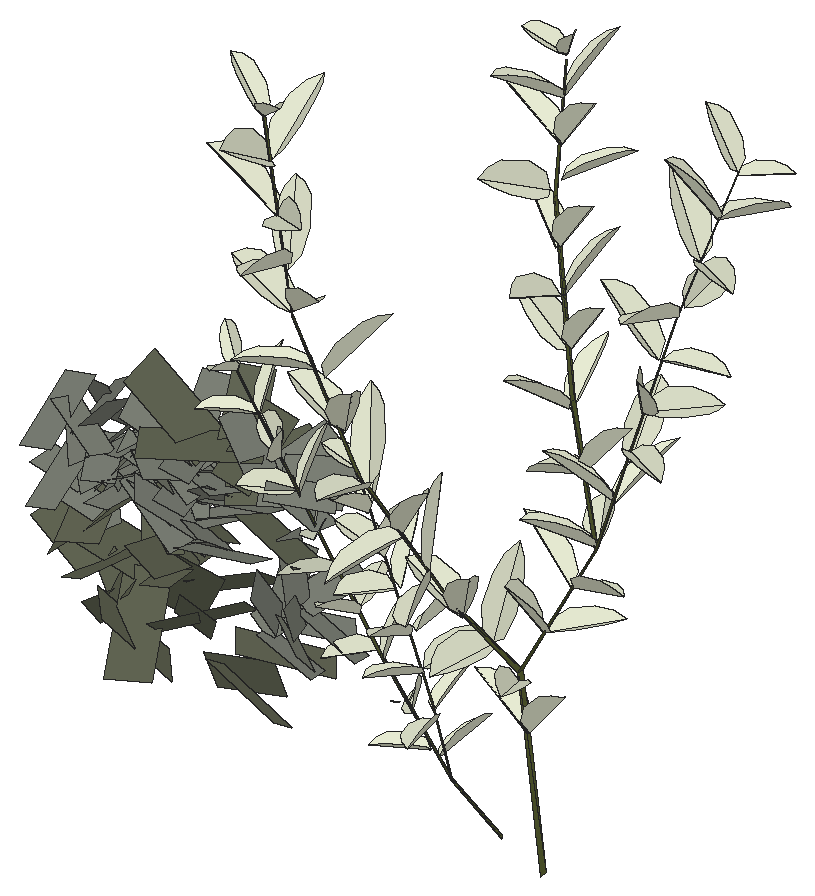
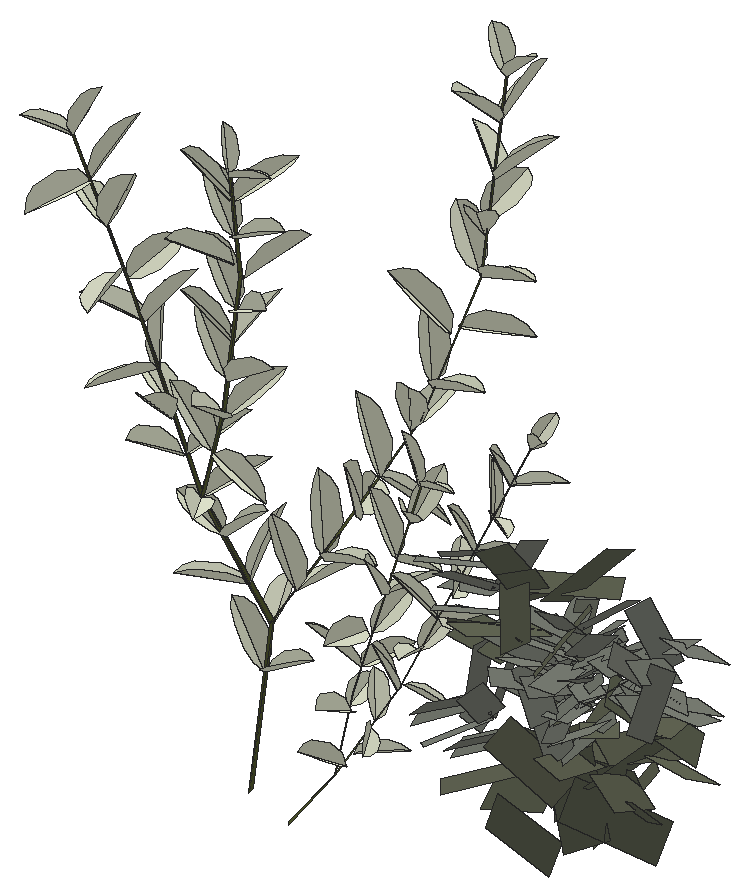
# SketchUp Ruby script. Lengths in inches.
U = 1.inch
M = Sketchup.active_model
def pt(a) = Geom::Point3d.new(a.map { |v| v * U })
def face(e, loops, mat)
  f = e.add_face(loops[0].map { |a| pt(a) })
  loops[1..].each { |l| e.add_face(l.map { |a| pt(a) }).erase! }
  f.material = f.back_material = mat if mat
  f
end
# faces: each face lists its corners as indices into pts; further lists are holes
def faces(e, pts, list, mat = nil) = list.each { |f| face(e, (f[0].is_a?(Array) ? f : [f]).map { |l| l.map { |i| pts[i] } }, mat) }
# xy, xz, yz: faces in a plane at the given z, y or x. An outline is a flat list of corners, or four numbers for a rectangle; further outlines are holes
def ring(l) = l.size == 4 ? [[l[0], l[1]], [l[2], l[1]], [l[2], l[3]], [l[0], l[3]]] : l.each_slice(2).to_a
def flat(e, list, mat, &to3) = list.each { |f| face(e, (f[0].is_a?(Array) ? f : [f]).map { |l| ring(l).map { |u, v| to3.(u, v) } }, mat) }
def xy(e, z, list, mat = nil) = flat(e, list, mat) { |x, y| [x, y, z] }
def xz(e, y, list, mat = nil) = flat(e, list, mat) { |x, z| [x, y, z] }
def yz(e, x, list, mat = nil) = flat(e, list, mat) { |y, z| [x, y, z] }
def lines(e, pts, list) = list.each { |a, b| e.add_line(pt(pts[a]), pt(pts[b])) }
# prism: a flat outline (further loops are holes) pulled along v
def prism(e, loops, v, mat = nil)
  f = face(e, loops, mat); d = Geom::Vector3d.new(v.map { |x| x * U })
  f.pushpull(f.normal.samedirection?(d) ? d.length : -d.length)
end
def box(e, o, s, mat = nil) = prism(e, [[o, [o[0] + s[0], o[1], o[2]], [o[0] + s[0], o[1] + s[1], o[2]], [o[0], o[1] + s[1], o[2]]]], [0, 0, s[2]], mat)
def at(x, y, z, deg = 0) = Geom::Transformation.translation(pt([x, y, z])) * Geom::Transformation.rotation(ORIGIN, Z_AXIS, deg.degrees)
def axes(o, x, y, z) = Geom::Transformation.new([*x, 0, *y, 0, *z, 0, *pt(o).to_a, 1])
def part(name) = M.definitions.add(name)
# library, detail: a bought-in or finely detailed component or shape, given as its bounding box
def library(name, o, s) = part(name).tap { |d| box(d.entities, o, s) }
def detail(e, o, s) = box(e.add_group.entities, o, s)
def put(e, d, t, mat = nil) = e.add_instance(d, t).tap { |i| i.material = mat if mat }
def group(e, t, mat = nil) = e.add_group.tap { |g| g.transformation = t; g.material = mat if mat }.entities
root = M.entities
M.materials.add("0ad16as01f6asdLeafVar1sfd015as60f1as6").color = [231, 235, 211]
M.materials.add("asdfasdf0165f6asdLeafVar1sfd015as60f1as6").color = [231, 235, 211]
M.materials.add("dw_stemssadfasdfa0sdf1s01d6w1").color = [90, 97, 50]
M.materials.add("viburnumblaasdfas0df1w06d").color = [98, 102, 84]
M.materials.add("viburnumbladsadfasdfad0w122").color = [125, 129, 119]
c1 = part("Component\#315")
p = [[0.25,0,0],[2.05,0.01,0.35],[1.81,4.2,1.66],[0,4.19,1.3125]]
faces(c1.entities,p,[[0,1,2,3]],"viburnumbladsadfasdfad0w122")
c2 = part("viburnumblad2")
put(c2.entities,c1,axes([-19.23,-4.49,-32.18],[83.35428,0,0],[0,79.38502,0],[0,0,83.35428]))
c3 = part("Component\#314")
p = [[0.14,0,0],[2.58,0.05,0.25],[2.44,5.11,2.64],[0,5.05,2.39]]
faces(c3.entities,p,[[0,1,2,3]],"viburnumblaasdfas0df1w06d")
c4 = part("viburnumblad1\#2")
put(c4.entities,c3,axes([-37.25,6.23,19.31],[75.98784,0,0],[0,65.50676,0],[0,0,75.98784]))
c5 = part("vdw_leaf\#1")
p = [[0,0,0],[-2.77,1.61,2.32],[-4.3125,6.1,4.5],[-3.97,13.49,6.09],[-2.47,18.57,6.3],[-0.2,22.73,5.75],
  [2.54,19.66,6.85],[4.3,15.93,7.09],[5.03,7.6,5.43],[3.32,1.76,2.74]]
faces(c5.entities,p,[[0,1,2,3,4,5],[0,5,6,7,8,9]],"0ad16as01f6asdLeafVar1sfd015as60f1as6")
c6 = part("dw_branch_3\#2")
p = [[-10.06,-1.6,62.9],[-0.2,1.54,-0.01],[-10.43,1.54,62.72],[0.18,-1.6,0.17],[-23.75,-21.66,88.91],[-25.7,-20.3,89.55],
  [13.4,11.62,104.56],[13.33,13.52,104.47],[-49.25,-41.87,130.3125],[-50.33,-40.21,130.71],[-4.97,21.13,143.98],[35.61,27.99,178.64],
  [-5.09,23.64,143.96],[35.32,29.14,178.46],[-67.7,-55.38,181.06],[-68.34,-54.45,181.62],[-22.8125,33.9,200.59],[-22.94,35.79,200.41],
  [56.61,36.78,229.75],[56.29,38.09,229.57],[-70.63,-67.46,248.85],[-70.72,-66.33,249.5],[-25.05,43.32,240.75],[-24.98,44.26,240.57]]
faces(c6.entities,p,[[0,1,2],[0,3,1],[4,2,5],[4,0,2],[6,0,2],[6,2,7],[8,4,5],[8,5,9],
  [10,6,7],[11,6,7],[10,7,12],[11,7,13],[14,8,9],[14,9,15],[16,10,12],[16,12,17],
  [18,11,13],[18,13,19],[20,14,15],[20,15,21],[22,16,17],[22,17,23]],"dw_stemssadfasdfa0sdf1s01d6w1")
c7 = part("dw_branch3\#2")
put(c7.entities,c5,axes([-70.33,-63.58,233.32],[-1.00752,0.412,0.78596],[-0.24851,-1.22189,0.32195],[0.83141,0.09817,1.01433]))
put(c7.entities,c5,axes([-66.93,-54.91,182.82],[-0.84976,-0.98359,0.33619],[0.99572,-0.74889,0.32577],[-0.05223,0.46521,1.22907]))
put(c7.entities,c5,axes([-46.12,-39.49,126.35],[1.23843,0.5364,0.23552],[-0.56438,0.94474,0.81599],[0.15707,-0.83465,1.07498]))
put(c7.entities,c5,axes([13.0625,13.13,104.77],[-1.01271,0.69982,-0.26884],[-0.74268,-0.99813,0.19939],[-0.10222,0.31872,1.21473]))
put(c7.entities,c5,axes([-18.87,30.42,186.42],[0.36309,1.06515,-0.56675],[-1.14134,0.49515,0.19939],[0.39128,0.45593,1.10754]))
put(c7.entities,c5,axes([-3.2,4.15,75.77],[-1.04153,0.55414,0.44243],[-0.23365,-1.01045,0.71554],[0.6695,0.50943,0.93801]))
put(c7.entities,c5,axes([23.2,19.41,136.3],[-0.65687,-1.11295,-0.05714],[1.05857,-0.61429,-0.20411],[0.15163,-0.1536,1.24868]))
put(c7.entities,c5,axes([-25.57,35.48,201.32],[-0.64726,0.62827,0.87973],[-0.71635,-1.0172,0.19939],[0.80962,-0.39773,0.87973]))
put(c7.entities,c5,axes([-36.37,-32.14,110.35],[-0.80747,1.09962,0.12544],[-0.83333,-0.50188,-0.96467],[-0.72833,-0.64487,0.96467]))
put(c7.entities,c5,axes([-9.89,26.72,156.79],[0.45529,1.02969,0.56572],[-1.16919,0.33753,0.32662],[0.11537,-0.64297,1.07744]))
put(c7.entities,c5,axes([-26.57,46.1,241.0625],[0.00015,0.80921,0.22536],[-0.83985,0.00446,-0.01542],[-0.01605,-0.22532,0.80906]))
put(c7.entities,c5,axes([-9.2,-2.58,61.06],[-1.10001,-0.40312,0.39014],[0.40883,-1.1116,0.00411],[0.35732,0.13566,1.14763]))
put(c7.entities,c5,axes([-69.91,-63.11,233.93],[1.36249,-0.1432,0],[0.13201,1.25603,0.5309],[-0.05549,-0.52799,1.26295]))
put(c7.entities,c5,axes([32.2,25.46,166.13],[0.06878,-1.29051,-0.05714],[1.22165,0.07415,-0.20411],[0.2113,-0.04403,1.24868]))
put(c7.entities,c5,axes([-5.68,-0.66,44.43],[-0.48448,-1.12287,0.17078],[0.98138,-0.33653,0.57135],[-0.48308,0.36756,1.04626]))
put(c7.entities,c5,axes([43.45,32.81,198.64],[0.5408,1.19584,0.14106],[-0.94242,0.32409,0.86557],[0.74952,-0.45533,0.98656]))
put(c7.entities,c5,axes([12.52,14.14,104.98],[1.02694,0.54888,0.41092],[-0.53566,1.05407,-0.06927],[-0.38969,-0.12321,1.13846]))
put(c7.entities,c5,axes([44.55,32.375,198.73],[-0.65687,-1.11295,-0.05714],[1.05857,-0.61429,-0.20411],[0.15163,-0.1536,1.24868]))
put(c7.entities,c5,axes([-5.67,21.17,141.44],[-1.10726,0.43603,-0.32953],[-0.49537,-1.03435,0.29588],[-0.17521,0.40597,1.12589]))
put(c7.entities,c5,axes([55.69,37.84,229.48],[0.18984,0.96334,0.18958],[-0.71996,0.0053,0.69399],[0.66755,-0.26823,0.69457]))
put(c7.entities,c5,axes([-21.52,36.85,205.2],[0.72606,-0.98817,0.14519],[0.94364,0.7084,0.10251],[-0.16885,0.05176,1.19664]))
put(c7.entities,c5,axes([-68.51,-56.35,196.07],[1.16319,0.72381,0],[-0.66725,1.0723,0.5309],[0.28049,-0.45075,1.26295]))
put(c7.entities,c6,at(0.01,-0.09,-0.02),"dw_stemssadfasdfa0sdf1s01d6w1")
put(c7.entities,c5,axes([-2.49,5.18,75.91],[0.78614,-0.90346,-0.30078],[0.86953,0.79562,-0.11715],[0.28546,-0.14014,1.16705]))
put(c7.entities,c5,axes([-23.125,-16.22,82.25],[0.32175,1.32576,0.12544],[-1.33153,0.31835,0.05068],[0.01989,-0.13382,1.3633]))
put(c7.entities,c5,axes([-23.75,41.99,230.3],[0.85958,-0.87451,0.14519],[0.66531,0.75721,0.62192],[-0.54076,-0.36226,1.01955]))
put(c7.entities,c5,axes([27.07,22.48,149.34],[0.92952,-0.64745,-0.62467],[0.50188,1.074,-0.36637],[0.71693,0.02135,1.04468]))
put(c7.entities,c5,axes([17.66,16.25,119.93],[-0.91649,0.83891,-0.3601],[-0.87434,-0.77966,0.40896],[0.0492,0.54447,1.14321]))
put(c7.entities,c5,axes([-68.37,-54.54,181.63],[0.32047,1.28399,0.35434],[-1.33153,0.31835,0.05068],[-0.03484,-0.35624,1.32241]))
put(c7.entities,c5,axes([-28.98,-27.1,96.48],[-0.8814,-0.35966,-0.98523],[0.75246,-1.11336,-0.26672],[-0.73065,-0.71272,0.91382]))
put(c7.entities,c5,axes([-15.23,28.43,172.72],[-1.21149,0.11898,0.32517],[-0.09739,-1.25259,0.09551],[0.33228,0.0667,1.21356]))
put(c7.entities,c5,axes([-17.5625,31.23,186.85],[-0.49275,-1.12287,0.14519],[0.95014,-0.33653,0.62192],[-0.53717,0.36756,1.01955]))
put(c7.entities,c5,axes([26.7,21.22,149.39],[-1.00104,0.22334,0.83093],[0.36894,-1.0402,0.72406],[0.77731,0.78134,0.72643]))
put(c7.entities,c5,axes([-31.125,-24.87,97.38],[0.75482,-0.86936,0.69068],[-0.00159,0.80023,1.00899],[-1.08766,-0.58016,0.45842]))
put(c7.entities,c5,axes([-71.21,-66.73,248.67],[0.25207,0.96771,0],[-0.8921,0.23237,0.38752],[0.375,-0.09768,0.92186]))
put(c7.entities,c5,axes([-24.11,41.05,229.55],[-1.11612,0.51924,-0.26884],[-0.56394,-1.10897,0.19939],[-0.15444,0.29694,1.21473]))
put(c7.entities,c5,axes([6.75,8.37,91.63],[-0.33418,-1.12287,0.39014],[1.13558,-0.33653,0.00411],[0.10478,0.36756,1.14763]))
put(c7.entities,c5,axes([-26,45.89,241.63],[-0.26986,-0.70824,-0.32129],[0.56818,-0.39091,0.38449],[-0.49365,-0.09775,0.63011]))
put(c7.entities,c5,axes([3.74,17.32,124.35],[0.22441,1.22913,-0.16274],[-1.07812,0.11178,-0.64246],[-0.61228,0.25367,1.07162]))
put(c7.entities,c5,axes([-5.44,22.27,140.88],[1.2203,0.00475,0.31374],[-0.097,1.20386,0.35905],[-0.29841,-0.37189,1.1663]))
put(c7.entities,c5,axes([-13.79,29.35,173.31],[0.83169,-0.90108,0.14519],[0.68877,0.73594,0.62192],[-0.55187,-0.34509,1.01955]))
put(c7.entities,c5,axes([-16.92,-7.26,72.98],[1.30647,0.30378,-0.27886],[0.07026,0.74892,1.14503],[0.40633,-1.10623,0.69861]))
put(c7.entities,c5,axes([4.8,17.55,125.22],[-0.25598,-1.17842,0.26559],[1.01553,-0.08455,0.60363],[-0.56975,0.35087,1.00767]))
put(c7.entities,c5,axes([5.3125,8.35,91.45],[0.00638,1.22913,-0.27714],[-1.16413,0.11178,0.46895],[0.48205,0.25367,1.13617]))
put(c7.entities,c5,axes([38.12,30.57,183.07],[1.12534,0.26182,-0.63833],[-0.46674,1.18829,-0.33545],[0.5081,0.51169,1.10563]))
put(c7.entities,c5,axes([-70.41,-60.38,214.47],[-0.41425,1.30587,0],[-1.20383,-0.38188,0.5309],[0.50605,0.16053,1.26295]))
put(c7.entities,c5,axes([37.03,28.75,180.67],[-1.12533,0.00102,-0.63799],[-0.00113,-1.2408,0],[-0.62497,0.00057,1.10237]))
put(c7.entities,c5,axes([30.71,25.35,165.96],[-0.1364,1.29314,0.22715],[-1.08768,-0.23921,0.70862],[0.73536,-0.11394,1.09026]))
put(c7.entities,c5,axes([-38.05,-30.84,110.67],[-0.31533,-1.27379,-0.2839],[1.018,-0.40311,0.67794],[-0.74394,-0.05723,1.08307]))
put(c7.entities,c5,axes([50.11,34.45,213.36],[-1.05669,0.74401,-0.05714],[-0.616,-0.82138,0.69675],[0.37221,0.60904,1.04705]))
put(c7.entities,c5,axes([-65.32,-58.78,200.07],[-1.14597,-0.19668,-0.6713],[0.21784,-1.26924,0],[-0.64812,-0.11124,1.139]))
put(c7.entities,c5,axes([-53.2,-43.37,143.59],[-0.72817,-1.09167,-0.2839],[0.82127,-0.72411,0.67794],[-0.71934,0.19815,1.08307]))
put(c7.entities,c5,axes([-61.1,-50.25,163.67],[-0.52887,1.19686,-0.30066],[-1.10762,-0.57104,-0.32484],[-0.42634,0.12264,1.23812]))
put(c7.entities,c5,axes([-54.12,-42.96,142.67],[0.32175,1.32576,0.12544],[-1.33153,0.31835,0.05068],[0.01989,-0.13382,1.3633]))
put(c7.entities,c5,axes([22.03,20.08,132.3],[1.17066,0.5058,-0.34078],[-0.35758,1.16671,0.50333],[0.49407,-0.35407,1.17172]))
put(c7.entities,c5,axes([-8.59,26.04,158.21],[-0.49275,-1.12287,0.14519],[0.95014,-0.33653,0.62192],[-0.53717,0.36756,1.01955]))
put(c7.entities,c5,axes([49.92,34.03,213.7],[1.24742,-0.35176,0.25024],[0.42127,1.159,-0.4708],[-0.09426,0.52477,1.20753]))
put(c7.entities,c5,axes([-70.34,-67.02,249.05],[-0.57048,-0.79684,0],[0.73827,-0.52855,0.24329],[-0.20203,0.14464,0.92729]))
put(c7.entities,c5,axes([56.04,36.81,228.63],[0.33451,-0.90845,-0.15237],[0.87636,0.33365,-0.06538],[0.11487,-0.11636,0.94597]))
put(c7.entities,c5,axes([-69.93,-60.58,214.88],[-0.45293,-0.99272,-0.78227],[1.14635,-0.58199,0.07483],[-0.40282,-0.65636,1.06615]))
put(c7.entities,c5,axes([-16.77,-8.59,72.7],[-1.22785,0.11509,0.53076],[-0.24879,-1.22495,-0.30991],[0.46742,-0.38989,1.16587]))
put(c7.entities,c5,axes([18.29,17.18,119.24],[1.19981,-0.45946,0.3029],[0.40159,1.22775,0.27158],[-0.37626,-0.1547,1.25575]))
put(c7.entities,c5,axes([-6.73,-0.68,43.74],[0.05346,1.22913,-0.27201],[-1.22696,0.11178,0.26396],[0.28163,0.25367,1.20164]))
put(c7.entities,c5,axes([-58.57,-48.42,160.98],[0.43385,-1.23789,0.39533],[1.04879,0.57965,0.66404],[-0.76727,0.09236,1.13122]))
put(c7.entities,c5,axes([-23.4,38.49,215.38],[0.06762,1.22913,-0.26884],[-1.23909,0.11178,0.19939],[0.21835,0.25367,1.21473]))
put(c7.entities,c5,axes([-22.21,-16.62,83.17],[-0.72817,-1.09167,-0.2839],[0.82127,-0.72411,0.67794],[-0.71934,0.19815,1.08307]))
put(c7.entities,c5,axes([-45.7,-40.77,126.53],[-1.33715,-0.0713,-0.0976],[0.07167,-1.28508,-0.04314],[-0.09306,-0.0492,1.31098]))
put(c7.entities,c5,axes([-22.39,38.51,216.12],[-0.49275,-1.12287,0.14519],[0.95014,-0.33653,0.62192],[-0.53717,0.36756,1.01955]))
c8 = part("vdw_leaf\#3")
p = [[0,0,0],[-2.77,1.61,2.32],[-4.3125,6.1,4.5],[-3.97,13.49,6.09],[-2.47,18.57,6.3],[-0.2,22.73,5.75],
  [2.54,19.66,6.85],[4.3,15.93,7.09],[5.03,7.6,5.43],[3.32,1.76,2.74]]
faces(c8.entities,p,[[0,1,2,3,4,5],[0,5,6,7,8,9]],"asdfasdf0165f6asdLeafVar1sfd015as60f1as6")
c9 = part("dw_brancj_2\#2")
p = [[9.7,-0.22,29.95],[0.23,-1.96,0.34],[-0.05,1.51,0.11],[9.65,1.51,29.46],[18.64,-8.75,84.43],[18.96,-6.63,84.625],
  [1.53,6.02,63.68],[1.42,8.18,63.25],[-10.58,8.77,161.17],[-10.41,9.98,160.68],[26.34,-9.37,211.72],[26.57,-8.28,211.23]]
faces(c9.entities,p,[[0,1,2],[0,2,3],[4,0,3],[4,3,5],[6,0,3],[6,3,7],[8,6,7],[8,7,9],
  [10,4,5],[10,5,11]],"dw_stemssadfasdfa0sdf1s01d6w1")
c10 = part("vdw_branch2\#3")
put(c10.entities,c8,axes([19.53,-5.9,102.42],[1.12377,-0.50004,0],[0.46097,1.03596,0.47664],[-0.19377,-0.43548,1.13389]))
put(c10.entities,c8,axes([-5.89,6.52,109.44],[-1.07209,0.83679,0],[-0.77141,-0.98832,0.52702],[0.32427,0.41545,1.25373]))
put(c10.entities,c8,axes([-0.44,8.23,75.28],[0.88709,-0.9947,0],[0.92159,0.82189,0.33087],[-0.25219,-0.22491,1.26111]))
put(c10.entities,c8,axes([24.71,-8.97,190.81],[-0.82641,0.91101,0],[-0.83983,-0.76184,0.47664],[0.35303,0.32025,1.13389]))
put(c10.entities,c8,axes([-2.29,8.24,91.35],[1.24603,-0.47303,0],[0.43826,1.15445,0.33087],[-0.11993,-0.31592,1.26111]))
put(c10.entities,c8,axes([12.26,-3.11,37.92],[-0.64625,1.02205,0.22511],[-1.04383,-0.61044,-0.22511],[-0.07533,-0.30931,1.18809]))
put(c10.entities,c8,axes([26.17,-9.17,210.27],[-0.99452,-0.10453,0],[0.09636,-0.91681,0.38752],[-0.04051,0.38539,0.92186]))
put(c10.entities,c8,axes([-6.07,9.4,125.35],[-0.90214,-0.98107,0],[0.90896,-0.83583,0.33087],[-0.24874,0.22873,1.26111]))
put(c10.entities,c8,axes([-4.13,7.29,110.58],[0.44715,-1.078,0.64369],[1.05816,0.63649,0.33087],[-0.58725,0.40856,1.09216]))
put(c10.entities,c8,axes([23.91,-8.22,171.96],[0.62307,0.85009,-0.63406],[-0.71531,0.8798,0.47664],[0.78296,0.12729,0.94004]))
put(c10.entities,c9,at(-0.09,0.18,-0.25),"dw_stemssadfasdfa0sdf1s01d6w1")
put(c10.entities,c8,axes([23.34,-9.65,156.59],[-0.31364,-1.00782,0.58216],[1.10369,-0.17062,0.29925],[-0.17137,0.6239,0.98776]))
put(c10.entities,c8,axes([15.03,-3.37,58.83],[-1.05425,-0.00194,0.58442],[-0.14303,-1.11707,-0.26172],[0.55355,-0.3046,0.99755]))
put(c10.entities,c8,axes([-11.625,9.46,160.37],[0.36812,0.92978,0],[-0.85713,0.33936,0.38752],[0.3603,-0.14265,0.92186]))
put(c10.entities,c8,axes([21.32,-8.53,138.72],[1.21379,0.19904,0],[-0.19904,1.21379,0],[0,0,1.23]))
put(c10.entities,c8,axes([22.54,-9.2,141.43],[-1.02887,0.17955,0.60182],[-0.23387,-1.13057,-0.06253],[0.56696,-0.17376,1.02111]))
put(c10.entities,c8,axes([23.9,-8.82,173.84],[-1.14567,-0.37474,0],[0.35918,-1.0981,0.04438],[-0.01409,0.04308,1.17993]))
put(c10.entities,c8,axes([-7.84,8.92,143.59],[-1.26971,0.40522,0],[-0.37543,-1.17638,0.33087],[0.10274,0.32192,1.26111]))
put(c10.entities,c8,axes([19.77,-8.01,85.98],[-0.32405,-1.14591,0.18674],[1.10278,-0.32969,-0.10948],[0.15845,0.14442,1.16117]))
put(c10.entities,c8,axes([-0.62,5.76,76.34],[-0.08879,1.17576,-0.67771],[-1.34525,-0.16582,-0.11144],[-0.17897,0.66309,1.17383]))
put(c10.entities,c8,axes([20.49,-8.22,121.07],[0.39924,-0.78471,-0.8233],[1.08735,0.33121,0.2116],[0.09035,-0.83005,0.83495]))
put(c10.entities,c8,axes([15.15,-3.72,62.9],[1.16251,0.40128,-0.0211],[-0.39924,1.16074,0.07874],[0.0456,-0.06757,1.2273]))
put(c10.entities,c8,axes([20.72,-8.08,120.26],[-0.03693,1.2277,-0.06551],[-1.22944,-0.03698,0],[-0.00197,0.06548,1.22825]))
put(c10.entities,c8,axes([22.58,-8.36,155.57],[-0.56247,1.09386,0],[-1.00839,-0.51852,0.47664],[0.42389,0.21796,1.13389]))
put(c10.entities,c8,axes([3.97,3.13,57.96],[-1.09459,0.76041,0],[-0.72262,-1.0402,-0.1735],[-0.10109,-0.14552,1.29352]))
put(c10.entities,c8,axes([-10.8,9.06,160.75],[-0.66334,-0.72138,0],[0.66835,-0.61458,0.24329],[-0.1829,0.16818,0.92729]))
put(c10.entities,c8,axes([19.06,-9.3125,103.96],[-1.01345,0.25553,-0.60051],[-0.2265,-1.12952,-0.09839],[-0.59598,0.03076,1.01889]))
put(c10.entities,c8,axes([18.07,-6.2,81.7],[-0.56247,1.09386,0],[-1.00839,-0.51852,0.47664],[0.42389,0.21796,1.13389]))
put(c10.entities,c8,axes([12.95,-0.39,43.31],[0.13044,-1.19832,0],[1.11025,0.12085,0.29925],[-0.30382,-0.03307,1.14057]))
put(c10.entities,c8,axes([2.28,8.28,56.18],[1.32413,-0.31027,0],[0.30923,1.31968,-0.11144],[0.02542,0.1085,1.35543]))
put(c10.entities,c8,axes([-7.55,9.96,143.07],[1.34251,-0.21744,0],[0.20045,1.23761,0.52702],[-0.08426,-0.52024,1.25373]))
put(c10.entities,c8,axes([26.15,-8.25,210.66],[0.94661,-0.25364,0],[0.235,0.87703,0.24329],[-0.06431,-0.24,0.92729]))
put(c10.entities,c8,axes([-6.48,11.37,125.16],[0.64635,1.10315,0.46356],[-1.16569,0.46153,0.52702],[0.27017,-0.6478,1.16488]))
put(c10.entities,c8,axes([25.74,-8.35,191.28],[0.13044,-1.19832,0],[1.11025,0.12085,0.29925],[-0.30382,-0.03307,1.14057]))
put(c10.entities,c8,axes([-5.125,7.47,91.6],[-1.10024,0.63688,0.48318],[-0.78682,-1.00808,-0.46292],[0.14137,-0.65404,1.184]))
put(root,c2,axes([2208.1,345.2,22.32],[0.00178,0.0105,0.00298],[-0.0098,0.00211,-0.00159],[-0.00226,-0.0026,0.01051]))
put(root,c2,axes([2214.56,346.86,22.69],[-0.00958,0.01044,0.00206],[-0.00856,-0.00879,0.00474],[0.00514,0.00211,0.0132]))
put(root,c4,axes([2210.52,344.04,12.65],[0.01503,0.00487,0.00033],[-0.00521,0.01551,0.00826],[0.00191,-0.00687,0.0141]))
put(root,c2,axes([2214.46,348.54,22.625],[-0.00988,-0.00976,0.00351],[0.01049,-0.01076,-0.00039],[0.00277,0.00219,0.01388]))
put(root,c2,axes([2220.76,345.66,29.29],[0.0022,-0.00655,-0.00816],[0.00813,0.00764,-0.00386],[0.00785,-0.0054,0.00541]))
put(root,c2,axes([2208.39,344.89,26.86],[0.00239,0.01136,-0.0048],[-0.01208,0.00314,0.00143],[0.00249,0.00434,0.01152]))
put(root,c2,axes([2203.84,344.05,26.41],[0.01523,-0.00004,0.00037],[-0.00005,0.01486,0.00338],[-0.00037,-0.00338,0.01485]))
put(root,c2,axes([2221.69,348.18,18.7],[-0.00745,0.00026,0.01011],[0.00262,-0.01208,0.00224],[0.00977,0.00344,0.00711]))
put(root,c2,axes([2214.05,348.625,27.04],[-0.01175,-0.00377,0.00233],[0.00341,-0.01191,-0.00208],[0.00284,-0.00132,0.01217]))
put(root,c4,axes([2207.1,343.9,18.21],[0.01155,-0.00606,0.00446],[0.00831,0.01316,-0.00362],[-0.00229,0.00493,0.01266]))
put(root,c4,axes([2211.09,345.44,28.48],[0.00835,-0.01477,-0.00252],[0.01522,0.00998,-0.00805],[0.00724,0.00145,0.01548]))
put(root,c4,axes([2212.09,347.49,11.87],[-0.01033,0.0106,0.00208],[-0.0106,-0.01173,0.00714],[0.00578,0.00298,0.01347]))
put(root,c2,axes([2220.34,347.16,18.08],[-0.00627,0.00896,0.00619],[-0.00305,-0.00837,0.00903],[0.01046,0.00298,0.00629]))
put(root,c4,axes([2205.0625,345.75,18.96],[0.0081,-0.01447,0.00211],[0.01627,0.00971,0.00411],[-0.00412,0.00005,0.0162]))
put(root,c2,axes([2204.25,344.09,22.59],[0.01462,-0.00004,0.00036],[-0.00005,0.01605,0.00365],[-0.00037,-0.00338,0.01485]))
put(root,c4,axes([2207.29,343.48,20.74],[0.01294,0.00473,-0.00003],[-0.00539,0.01473,-0.00308],[-0.00088,0.0025,0.01352]))
put(root,c2,axes([2208.03,346.15,24.61],[0.007,-0.00987,0.00339],[0.00957,0.00618,-0.0018],[-0.00027,0.0039,0.01194]))
put(root,c4,axes([2212.21,349.72,18.8],[-0.01223,0.00026,0.00635],[-0.0009,-0.01592,-0.0011],[0.0063,-0.0012,0.0122]))
put(root,c4,axes([2214.9,346.71,27.32],[0.00084,0.01421,0.00442],[-0.01582,-0.0012,0.00687],[0.00595,-0.00438,0.01294]))
put(root,c2,axes([2207.41,346.75,23.98],[0.00604,-0.00926,0.00001],[0.00806,0.00526,0.00544],[-0.00456,-0.00296,0.00963]))
put(root,c2,axes([2206.28,348.02,26.51],[-0.00259,-0.01229,0.00001],[0.0107,-0.00225,0.00618],[-0.00604,0.00128,0.01094]))
put(root,c2,axes([2207.69,345.23,23.43],[0.01283,-0.0027,-0.00001],[0.00224,0.01066,-0.00301],[0.0007,0.00327,0.01211]))
put(root,c2,axes([2213.5,348.31,25.38],[-0.01046,0.00558,0.00416],[-0.00525,-0.01025,0.00054],[0.00396,-0.00141,0.01184]))
put(root,c2,axes([2213.14,349.08,24.1],[-0.01227,-0.00394,0.00243],[0.00307,-0.01072,-0.00188],[0.00284,-0.00132,0.01217]))
put(root,c2,axes([2213.23,347.73,24.05],[-0.00945,0.00658,-0.00199],[-0.00667,-0.00798,0.00533],[0.00164,0.00544,0.01021]))
put(root,c2,axes([2207.86,344.8,25.19],[0.01038,0.0062,-0.0034],[-0.00717,0.01088,-0.00204],[0.00185,0.00346,0.01194]))
put(root,c2,axes([2206.5,345.88,23.43],[0.0027,0.01283,-0.00001],[-0.01066,0.00224,-0.00301],[-0.00327,0.0007,0.01211]))
put(root,c4,axes([2207.83,345.29,18.21],[0.00606,0.01155,0.00446],[-0.01316,0.00831,-0.00362],[-0.00493,-0.00229,0.01266]))
put(root,c2,axes([2220.11,348.91,17.86],[-0.00427,-0.00859,0.00811],[0.00683,-0.00794,-0.00482],[0.00917,0.00302,0.00803]))
put(root,c7,axes([2237.59,349.42,7.47],[0.1634,0,0],[0,0.1634,0],[0,0,0.20106]))
put(root,c2,axes([2218.99,346.3,27.52],[0.00288,0.01252,0.00147],[-0.00904,0.00098,0.00938],[0.00888,-0.00309,0.00888]))
put(root,c2,axes([2206.97,345.5,23.55],[0.00856,0.00558,0.00422],[-0.00642,0.00891,0.00123],[-0.00278,-0.00341,0.01014]))
put(root,c10,axes([2233.09,351.22,7.57],[-0.10096,-0.0593,-0.07152],[0.0662,-0.11272,0],[-0.05012,-0.02944,0.14408]))
put(root,c4,axes([2214.76,348.28,13.64],[0.00066,-0.01186,0.00699],[0.01121,-0.00532,-0.01007],[0.0098,0.00532,0.0081]))
put(root,c2,axes([2219.59,348.5,27.68],[-0.00288,-0.01252,-0.00147],[0.01138,-0.00177,-0.00721],[0.00645,-0.00276,0.01087]))
put(root,c2,axes([2213.59,348.83,25.17],[-0.01151,-0.00142,0.00146],[0.00195,-0.0101,0.00555],[0.00059,0.0057,0.01018]))
put(root,c2,axes([2213.1,346.35,21.51],[-0.00037,0.01298,-0.00224],[-0.01317,0.00059,0.00559],[0.0056,0.0024,0.01296]))
put(root,c2,axes([2213.06,347.39,27.02],[-0.00304,0.01166,0.00355],[-0.01127,-0.00408,0.00376],[0.00464,-0.00228,0.01145]))
put(root,c4,axes([2211.57,346.68,15.05],[0.00317,-0.01127,0.00742],[0.01555,0.00409,-0.00043],[-0.00159,0.00725,0.0117]))
put(root,c4,axes([2217.09,349.46,23.67],[-0.00406,-0.01328,0.00293],[0.01275,-0.00581,-0.00863],[0.008,0.00014,0.01172]))
put(root,c2,axes([2207.77,345.96,21.07],[0.0081,0.00545,0.00286],[-0.00642,0.00891,0.00123],[-0.00184,-0.00279,0.01054]))
put(root,c2,axes([2213.13,348.68,21.19],[-0.0002,-0.01371,0.00098],[0.01527,-0.0004,-0.00242],[0.00226,0.00098,0.01411]))
put(root,c4,axes([2212.73,349.65,13.95],[-0.01191,-0.00399,0.00577],[0.00688,-0.0137,0.00471],[0.00376,0.00597,0.01189]))
put(root,c2,axes([2212.55,347.05,22.8125],[-0.00179,0.01029,-0.00409],[-0.01223,-0.00094,0.00298],[0.00221,0.00457,0.01052]))
put(root,c2,axes([2213.21,349.11,23.47],[-0.00682,-0.00858,0.00405],[0.00958,-0.00605,0.00332],[-0.00034,0.0052,0.01046]))
put(root,c2,axes([2213.98,346.7,24.8125],[0.00021,0.01428,-0.00102],[-0.01317,0.00059,0.00559],[0.00561,0.00086,0.01315]))
put(root,c4,axes([2216.34,346.25,27.16],[0.01029,0.00428,-0.00658],[0.00078,0.01194,0.00879],[0.00737,-0.00649,0.00685]))
put(root,c2,axes([2213.04,349.64,25.83],[-0.00616,-0.01091,-0.00086],[0.01132,-0.00616,-0.00282],[0.00193,-0.00206,0.01224]))
put(root,c2,axes([2207.24,346.5,22.34],[0.01032,-0.0026,0.00299],[0.00135,0.01024,0.00424],[-0.00373,-0.00356,0.00978]))
put(root,c4,axes([2210.57,349.02,16.32],[-0.00358,0.0126,0.00711],[-0.01496,-0.00708,0.005],[0.00656,-0.00511,0.01237]))
put(root,c4,axes([2212.2,350.37,21.29],[-0.00859,-0.01039,0.00287],[0.01161,-0.0105,-0.00325],[0.004,0.00034,0.01318]))
put(root,c2,axes([2212.37,347.97,24.15],[-0.00324,0.01089,0.00211],[-0.01127,-0.00408,0.00376],[0.00428,-0.00101,0.01177]))
put(root,c2,axes([2218.66,348.83,17.35],[0.00148,-0.01296,0.00142],[0.00776,-0.00002,-0.00823],[0.00903,0.00196,0.00851]))
put(root,c2,axes([2207.74,346.25,26.37],[0.01229,-0.00259,-0.00001],[0.00249,0.01185,-0.00335],[0.0007,0.00327,0.01211]))
put(root,c2,axes([2205.58,346.22,24.61],[0.00987,0.007,0.00339],[-0.00618,0.00957,-0.0018],[-0.0039,-0.00027,0.01194]))
put(root,c2,axes([2214.4375,349.2,24.51],[-0.00021,-0.01428,0.00102],[0.01414,-0.00037,-0.00224],[0.00226,0.00098,0.01411]))
put(root,c2,axes([2221.03,347.3,19.84],[-0.00141,0.01241,-0.00136],[-0.00618,0.00049,0.01093],[0.01085,0.0019,0.00605]))
put(root,c2,axes([2205.9375,347.95,24.65],[0.0062,-0.01038,0.0034],[0.00931,0.00714,0.00482],[-0.00586,0.00014,0.01111]))
put(root,c2,axes([2220.05,348.16,29.4],[0.00501,-0.0098,-0.00679],[0.00996,0.00749,-0.00346],[0.00656,-0.00389,0.01045]))
put(root,c2,axes([2212.29,348.85,22.23],[0.00176,-0.01022,0.00282],[0.01152,0.00195,-0.00013],[-0.00039,0.00304,0.01127]))
put(root,c2,axes([2212.54,347.9,25.63],[-0.00186,0.01072,-0.00426],[-0.01132,-0.00087,0.00276],[0.00221,0.00457,0.01052]))
put(root,c2,axes([2221.01,349.48,19.29],[0.00141,-0.01241,0.00136],[0.00862,-0.00002,-0.00914],[0.00903,0.00196,0.00851]))
put(root,c4,axes([2209.54,347.02,14.24],[0.00865,0.00658,0.00734],[-0.00992,0.01145,0.00143],[-0.0049,-0.0056,0.0108]))
put(root,c2,axes([2205.93,347.09,23.2],[0.01089,-0.00213,0.00325],[0.002,0.01232,0.0014],[-0.00372,-0.00076,0.01198]))
put(root,c4,axes([2211.29,346.33,20.05],[0.00989,0.00806,-0.00127],[-0.00946,0.01134,-0.00169],[0.00005,0.00193,0.01267]))
put(root,c2,axes([2218.01,348.51,26.87],[0.00481,-0.00941,-0.00652],[0.01076,0.00809,-0.00374],[0.00656,-0.00389,0.01045]))
put(root,c2,axes([2204.92,347.375,26.02],[0.01136,-0.00239,0.0048],[0.002,0.01232,0.0014],[-0.00498,-0.0005,0.01153]))
put(root,c2,axes([2212.88,349.56,27.58],[0.00304,-0.01166,-0.00355],[0.01206,0.00341,-0.00087],[0.00178,-0.0032,0.01202]))
put(root,c2,axes([2211.85,347.77,25.74],[0.00616,0.01091,0.00086],[-0.01009,0.00525,0.00563],[0.00448,-0.00342,0.01123]))
put(root,c2,axes([2212.625,346.9375,23.29],[0.00988,0.00976,-0.00351],[-0.00912,0.01058,0.00376],[0.00511,-0.00035,0.01338]))
put(root,c4,axes([2208.21,346.52,15.44],[0.01224,-0.00166,0.00834],[0.00122,0.01717,0.00163],[-0.00844,-0.00056,0.01227]))
put(root,c4,axes([2215.07,348.42,26.12],[0.00626,-0.00918,-0.00848],[0.01094,0.01129,-0.00412],[0.00772,-0.00395,0.00939]))
put(root,c2,axes([2212.69,349.96,19.59],[-0.0083,0.00785,-0.00197],[-0.00857,-0.00783,0.00492],[0.002,0.00498,0.01141]))
put(root,c2,axes([2218.53,347.7,28.3],[0.00997,-0.00134,-0.00814],[0.0038,0.01207,0.00267],[0.00731,-0.00445,0.00969]))
put(root,c4,axes([2210.7,346.64,17.76],[0.01241,-0.00186,0.00262],[0.00291,0.01409,-0.00376],[-0.00201,0.00365,0.01212]))
put(root,c2,axes([2219.37,347.4375,19.34],[0.00427,0.00859,-0.00811],[-0.005,0.00913,0.00703],[0.0107,0.00084,0.00653]))
put(root,c4,axes([2215.76,348.38,16],[0.00753,-0.01126,-0.00255],[0.00884,0.00827,-0.01044],[0.00867,0.00351,0.01012]))
put(root,c2,axes([2212.85,351.23,19.14],[-0.00925,-0.00862,0.00362],[0.00803,-0.00772,0.00213],[0.00081,0.00412,0.01188]))
put(root,c2,axes([2211.91,347.66,24.15],[0.00682,0.00858,-0.00405],[-0.00975,0.00742,-0.00069],[0.00196,0.0036,0.01094]))
put(root,c4,axes([2215.85,347.25,28.07],[0.00971,0.0077,-0.00377],[-0.00736,0.01191,0.00523],[0.00557,-0.00177,0.01033]))
put(root,c4,axes([2205.97,348.26,13.05],[0.00095,-0.01143,0.01095],[0.01752,0.00456,0.00324],[-0.00472,0.01026,0.01113]))
put(root,c2,axes([2212.5625,349.83,24.84],[0.00186,-0.01072,0.00426],[0.01152,0.00195,-0.00013],[-0.00059,0.00423,0.01088]))
put(root,c2,axes([2212.92,348.74,23.09],[0.00958,-0.01044,-0.00206],[0.01029,0.0098,-0.00181],[0.00273,-0.00027,0.01406]))
put(root,c2,axes([2213.28,351.18,20.62],[-0.01246,0.00054,0.00182],[0.00014,-0.01079,0.00417],[0.00189,0.00451,0.01162]))
put(root,c2,axes([2211.87,349.92,24.6],[0.00292,-0.01119,-0.00341],[0.01302,0.00368,-0.00094],[0.00178,-0.0032,0.01202]))
put(root,c2,axes([2219.26,348.83,19.07],[0.00627,-0.00896,-0.00619],[0.00573,0.0092,-0.00751],[0.00942,0.00088,0.00827]))
put(root,c4,axes([2210.36,351.51,13.21],[-0.01405,-0.00766,0.00571],[0.01107,-0.01374,0.00878],[0.00057,0.00947,0.0141]))
put(root,c2,axes([2211.43,347.99,22.55],[0.01201,0.00148,-0.00152],[-0.00157,0.01006,-0.00263],[0.00104,0.00309,0.01122]))
put(root,c2,axes([2211.59,348.9,23.65],[0.00945,-0.00658,0.00199],[0.00631,0.00831,-0.00248],[-0.00002,0.00335,0.01119]))
put(root,c2,axes([2218.02,347.83,18.42],[0.00716,-0.00025,-0.0097],[-0.0002,0.01356,-0.00049],[0.01011,0.00042,0.00745]))
put(root,c4,axes([2212.73,350.29,10.77],[-0.00376,-0.0039,0.01194],[0.01323,-0.00731,0.00178],[0.00528,0.01082,0.0052]))
put(root,c4,axes([2213.59,351.3,24.69],[-0.00832,0.00937,0.00389],[-0.0091,-0.01059,0.00604],[0.00643,0.00098,0.01139]))
put(root,c2,axes([2213.03,350.72,22.49],[-0.00876,0.00902,-0.0009],[-0.00857,-0.00783,0.00492],[0.00296,0.00403,0.01157]))
put(root,c2,axes([2211.89,348.32,27.56],[0.01175,0.00377,-0.00233],[-0.00262,0.01124,0.00497],[0.00358,-0.00416,0.0113]))
put(root,c4,axes([2211.95,350.9375,16.04],[-0.00313,-0.01186,0.00638],[0.01559,-0.00367,0.00082],[0.00085,0.00636,0.01225]))
put(root,c2,axes([2213.3,352.23,22.07],[-0.00886,-0.00826,0.00347],[0.00892,-0.00858,0.00237],[0.00081,0.00412,0.01188]))
put(root,c2,axes([2213,348.21,24.99],[0.01376,-0.00048,-0.00394],[0.00069,0.01429,0.00066],[0.00391,-0.00082,0.01375]))
put(root,c2,axes([2211.69,349.32,26.16],[0.01046,-0.00558,-0.00416],[0.00651,0.0105,0.0023],[0.00246,-0.00407,0.01163]))
put(root,c2,axes([2220.34,348.6,20.4375],[0.00745,-0.00026,-0.01011],[-0.00018,0.01255,-0.00046],[0.01011,0.00042,0.00745]))
put(root,c4,axes([2214.45,348.51,26.14],[0.01206,-0.00628,-0.00336],[0.00668,0.01448,-0.00311],[0.00388,0.00091,0.01211]))
put(root,c2,axes([2211.51,348.9,25.3],[0.01151,0.00142,-0.00146],[-0.00175,0.01118,-0.00292],[0.00104,0.00309,0.01122]))
put(root,c4,axes([2214.4375,352.9375,26.65],[-0.01002,-0.00367,0.00577],[0.0058,-0.01266,0.00203],[0.00466,0.00382,0.01053]))
put(root,c2,axes([2205.47,352.48,24.34],[-0.01322,-0.00136,-0.00142],[0.00017,-0.01043,0.00835],[-0.00196,0.00824,0.01034]))
put(root,c2,axes([2212.04,350.03,21.15],[0.00007,0.01222,-0.00309],[-0.01226,0.00091,0.00331],[0.0034,0.00296,0.01177]))
